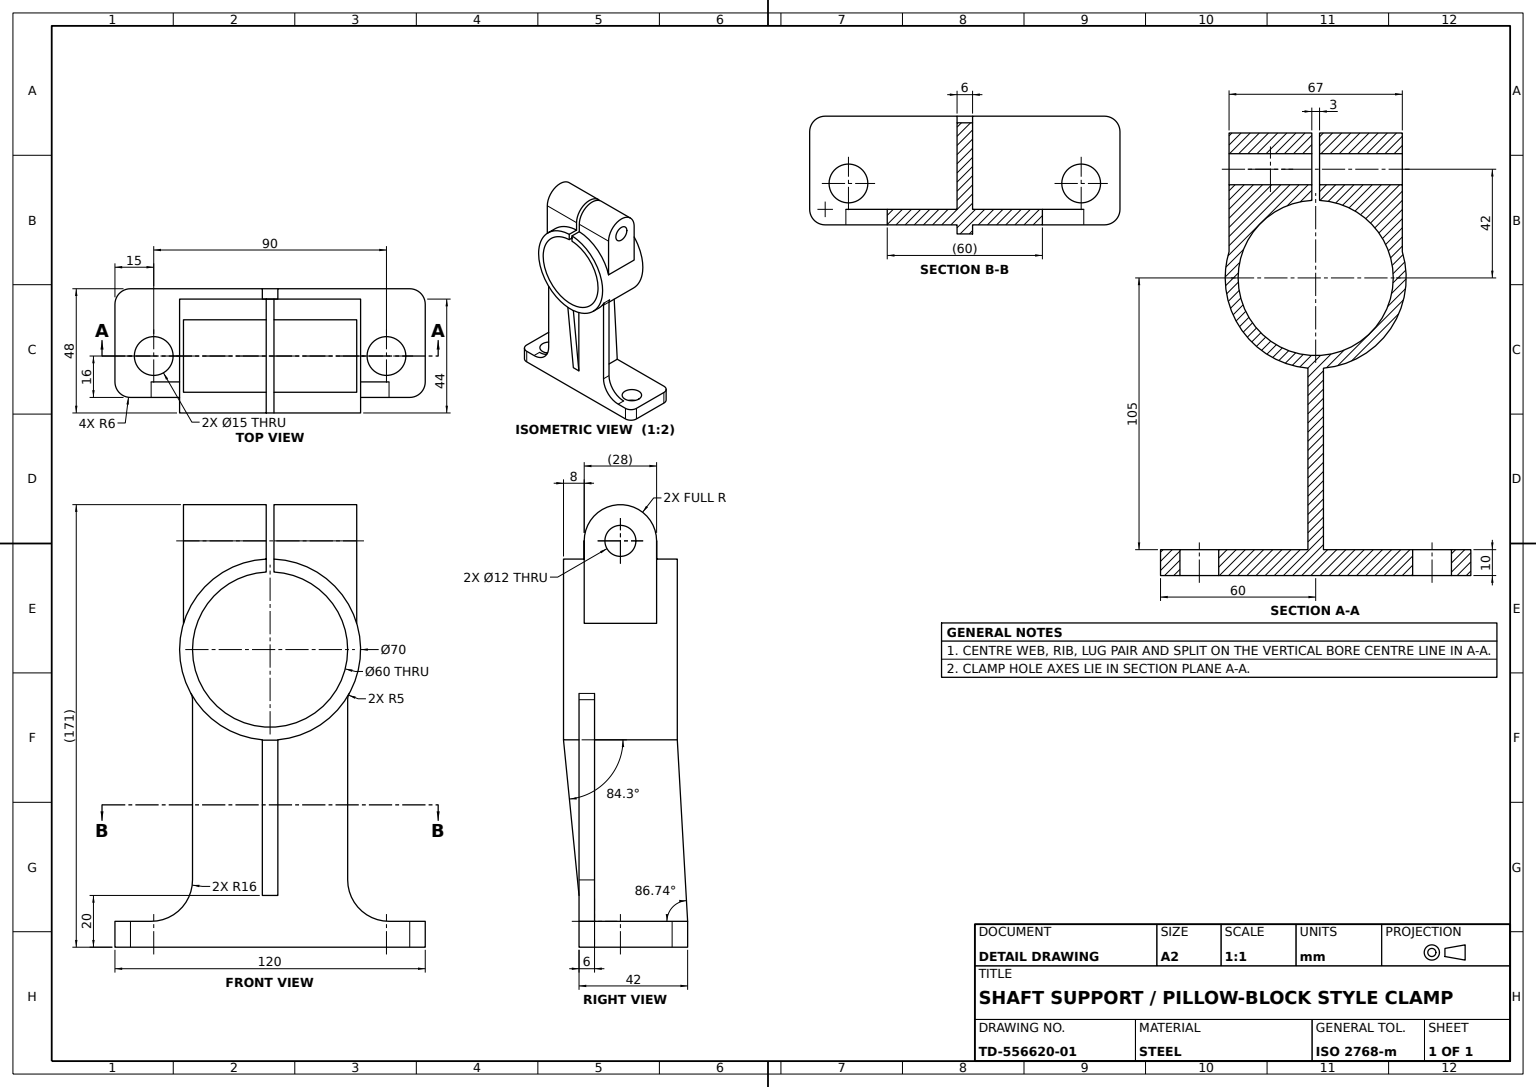
ISO-10303-21;
HEADER;
FILE_DESCRIPTION((''),'2;1');
FILE_NAME('','',(''),(''),'','','');
FILE_SCHEMA(('AUTOMOTIVE_DESIGN'));
ENDSEC;
DATA;
#1=APPLICATION_CONTEXT('');
#2=PRODUCT_CONTEXT('',#1,'mechanical');
#3=PRODUCT('','','',(#2));
#4=PRODUCT_DEFINITION_FORMATION('','',#3);
#5=PRODUCT_DEFINITION_CONTEXT('',#1,'design');
#6=PRODUCT_DEFINITION('','',#4,#5);
#7=PRODUCT_DEFINITION_SHAPE('','',#6);
#8=(LENGTH_UNIT()NAMED_UNIT(*)SI_UNIT(.MILLI.,.METRE.));
#9=(NAMED_UNIT(*)PLANE_ANGLE_UNIT()SI_UNIT($,.RADIAN.));
#10=(NAMED_UNIT(*)SI_UNIT($,.STERADIAN.)SOLID_ANGLE_UNIT());
#11=UNCERTAINTY_MEASURE_WITH_UNIT(LENGTH_MEASURE(1.E-05),#8,'distance_accuracy_value','');
#12=(GEOMETRIC_REPRESENTATION_CONTEXT(3)GLOBAL_UNCERTAINTY_ASSIGNED_CONTEXT((#11))GLOBAL_UNIT_ASSIGNED_CONTEXT((#8,#9,#10))REPRESENTATION_CONTEXT('',''));
#13=CARTESIAN_POINT('',(14.,34.967842,-1.5));
#14=VERTEX_POINT('',#13);
#15=CARTESIAN_POINT('',(22.,34.967842,-1.5));
#16=VERTEX_POINT('',#15);
#17=DIRECTION('',(1.,0.,0.));
#18=VECTOR('',#17,1000.);
#19=LINE('',#15,#18);
#20=EDGE_CURVE('',#14,#16,#19,.T.);
#21=ORIENTED_EDGE('',*,*,#20,.T.);
#22=CARTESIAN_POINT('',(22.,-34.871192,-3.));
#23=VERTEX_POINT('',#22);
#24=CARTESIAN_POINT('',(22.,0.,0.));
#25=DIRECTION('',(0.,0.,-1.));
#26=AXIS2_PLACEMENT_3D('',#24,#17,#25);
#27=CIRCLE('',#26,35.);
#28=EDGE_CURVE('',#23,#16,#27,.T.);
#29=ORIENTED_EDGE('',*,*,#28,.F.);
#30=CARTESIAN_POINT('',(16.,-34.871192,-3.));
#31=VERTEX_POINT('',#30);
#32=LINE('',#22,#18);
#33=EDGE_CURVE('',#31,#23,#32,.T.);
#34=ORIENTED_EDGE('',*,*,#33,.F.);
#35=CARTESIAN_POINT('',(16.,-16.944302,-30.625));
#36=VERTEX_POINT('',#35);
#37=CARTESIAN_POINT('',(16.,0.,0.));
#38=DIRECTION('',(-1.,0.,0.));
#39=AXIS2_PLACEMENT_3D('',#37,#38,#25);
#40=CIRCLE('',#39,35.);
#41=EDGE_CURVE('',#36,#31,#40,.T.);
#42=ORIENTED_EDGE('',*,*,#41,.F.);
#43=CARTESIAN_POINT('',(10.,-16.944302,-30.625));
#44=VERTEX_POINT('',#43);
#45=CARTESIAN_POINT('',(22.,-16.944302,-30.625));
#46=VECTOR('',#38,1000.);
#47=LINE('',#45,#46);
#48=EDGE_CURVE('',#36,#44,#47,.T.);
#49=ORIENTED_EDGE('',*,*,#48,.T.);
#50=CARTESIAN_POINT('',(10.,-34.871192,-3.));
#51=VERTEX_POINT('',#50);
#52=CARTESIAN_POINT('',(10.,0.,0.));
#53=AXIS2_PLACEMENT_3D('',#52,#38,#25);
#54=CIRCLE('',#53,35.);
#55=EDGE_CURVE('',#44,#51,#54,.T.);
#56=ORIENTED_EDGE('',*,*,#55,.T.);
#57=CARTESIAN_POINT('',(-22.,-34.871192,-3.));
#58=VERTEX_POINT('',#57);
#59=CARTESIAN_POINT('',(22.002,-34.871192,-3.));
#60=LINE('',#59,#46);
#61=EDGE_CURVE('',#51,#58,#60,.T.);
#62=ORIENTED_EDGE('',*,*,#61,.T.);
#63=CARTESIAN_POINT('',(-22.,34.967842,-1.5));
#64=VERTEX_POINT('',#63);
#65=CARTESIAN_POINT('',(-22.,0.,0.));
#66=AXIS2_PLACEMENT_3D('',#65,#17,#25);
#67=CIRCLE('',#66,35.);
#68=EDGE_CURVE('',#58,#64,#67,.T.);
#69=ORIENTED_EDGE('',*,*,#68,.T.);
#70=CARTESIAN_POINT('',(-14.,34.967842,-1.5));
#71=VERTEX_POINT('',#70);
#72=EDGE_CURVE('',#64,#71,#19,.T.);
#73=ORIENTED_EDGE('',*,*,#72,.T.);
#74=CARTESIAN_POINT('',(-14.,10.136567,-33.5));
#75=VERTEX_POINT('',#74);
#76=CARTESIAN_POINT('',(-14.,0.,0.));
#77=DIRECTION('',(0.,1.,0.));
#78=AXIS2_PLACEMENT_3D('',#76,#17,#77);
#79=CIRCLE('',#78,35.);
#80=EDGE_CURVE('',#75,#71,#79,.T.);
#81=ORIENTED_EDGE('',*,*,#80,.F.);
#82=CARTESIAN_POINT('',(14.,10.136567,-33.5));
#83=VERTEX_POINT('',#82);
#84=CARTESIAN_POINT('',(22.,10.136567,-33.5));
#85=LINE('',#84,#46);
#86=EDGE_CURVE('',#83,#75,#85,.T.);
#87=ORIENTED_EDGE('',*,*,#86,.F.);
#88=CARTESIAN_POINT('',(14.,0.,0.));
#89=DIRECTION('',(0.,0.,1.));
#90=AXIS2_PLACEMENT_3D('',#88,#38,#89);
#91=CIRCLE('',#90,35.);
#92=EDGE_CURVE('',#14,#83,#91,.T.);
#93=ORIENTED_EDGE('',*,*,#92,.F.);
#94=EDGE_LOOP('',(#21,#29,#34,#42,#49,#56,#62,#69,#73,#81,#87,#93));
#95=FACE_OUTER_BOUND('',#94,.T.);
#96=AXIS2_PLACEMENT_3D('',#24,#38,#89);
#97=CYLINDRICAL_SURFACE('',#96,35.);
#98=ADVANCED_FACE('',(#95),#97,.T.);
#99=CARTESIAN_POINT('',(0.,-115.,37.5));
#100=VERTEX_POINT('',#99);
#101=CARTESIAN_POINT('',(0.,-115.,52.5));
#102=VERTEX_POINT('',#101);
#103=CARTESIAN_POINT('',(0.,-115.,45.));
#104=DIRECTION('',(0.,-1.,0.));
#105=AXIS2_PLACEMENT_3D('',#103,#104,#89);
#106=CIRCLE('',#105,7.5);
#107=EDGE_CURVE('',#100,#102,#106,.T.);
#108=ORIENTED_EDGE('',*,*,#107,.F.);
#109=EDGE_CURVE('',#102,#100,#106,.T.);
#110=ORIENTED_EDGE('',*,*,#109,.F.);
#111=EDGE_LOOP('',(#108,#110));
#112=FACE_BOUND('',#111,.T.);
#113=CARTESIAN_POINT('',(-20.,-115.,60.));
#114=VERTEX_POINT('',#113);
#115=CARTESIAN_POINT('',(-26.,-115.,54.));
#116=VERTEX_POINT('',#115);
#117=CARTESIAN_POINT('',(-20.,-115.,54.));
#118=AXIS2_PLACEMENT_3D('',#117,#104,#89);
#119=CIRCLE('',#118,6.);
#120=EDGE_CURVE('',#114,#116,#119,.T.);
#121=ORIENTED_EDGE('',*,*,#120,.T.);
#122=CARTESIAN_POINT('',(-26.,-115.,-54.));
#123=VERTEX_POINT('',#122);
#124=CARTESIAN_POINT('',(-26.,-115.,-60.));
#125=VECTOR('',#89,1000.);
#126=LINE('',#124,#125);
#127=EDGE_CURVE('',#123,#116,#126,.T.);
#128=ORIENTED_EDGE('',*,*,#127,.F.);
#129=CARTESIAN_POINT('',(-20.,-115.,-60.));
#130=VERTEX_POINT('',#129);
#131=CARTESIAN_POINT('',(-20.,-115.,-54.));
#132=AXIS2_PLACEMENT_3D('',#131,#104,#89);
#133=CIRCLE('',#132,6.);
#134=EDGE_CURVE('',#123,#130,#133,.T.);
#135=ORIENTED_EDGE('',*,*,#134,.T.);
#136=CARTESIAN_POINT('',(10.,-115.,-60.));
#137=VERTEX_POINT('',#136);
#138=LINE('',#124,#46);
#139=EDGE_CURVE('',#137,#130,#138,.T.);
#140=ORIENTED_EDGE('',*,*,#139,.F.);
#141=CARTESIAN_POINT('',(16.,-115.,-54.));
#142=VERTEX_POINT('',#141);
#143=CARTESIAN_POINT('',(10.,-115.,-54.));
#144=AXIS2_PLACEMENT_3D('',#143,#104,#89);
#145=CIRCLE('',#144,6.);
#146=EDGE_CURVE('',#137,#142,#145,.T.);
#147=ORIENTED_EDGE('',*,*,#146,.T.);
#148=CARTESIAN_POINT('',(16.,-115.,54.));
#149=VERTEX_POINT('',#148);
#150=CARTESIAN_POINT('',(16.,-115.,-60.));
#151=VECTOR('',#25,1000.);
#152=LINE('',#150,#151);
#153=EDGE_CURVE('',#149,#142,#152,.T.);
#154=ORIENTED_EDGE('',*,*,#153,.F.);
#155=CARTESIAN_POINT('',(10.,-115.,60.));
#156=VERTEX_POINT('',#155);
#157=CARTESIAN_POINT('',(10.,-115.,54.));
#158=AXIS2_PLACEMENT_3D('',#157,#104,#89);
#159=CIRCLE('',#158,6.);
#160=EDGE_CURVE('',#149,#156,#159,.T.);
#161=ORIENTED_EDGE('',*,*,#160,.T.);
#162=CARTESIAN_POINT('',(-26.,-115.,60.));
#163=LINE('',#162,#18);
#164=EDGE_CURVE('',#114,#156,#163,.T.);
#165=ORIENTED_EDGE('',*,*,#164,.F.);
#166=EDGE_LOOP('',(#121,#128,#135,#140,#147,#154,#161,#165));
#167=FACE_OUTER_BOUND('',#166,.T.);
#168=CARTESIAN_POINT('',(0.,-115.,-37.5));
#169=VERTEX_POINT('',#168);
#170=CARTESIAN_POINT('',(0.,-115.,-52.5));
#171=VERTEX_POINT('',#170);
#172=CARTESIAN_POINT('',(0.,-115.,-45.));
#173=AXIS2_PLACEMENT_3D('',#172,#104,#89);
#174=CIRCLE('',#173,7.5);
#175=EDGE_CURVE('',#169,#171,#174,.T.);
#176=ORIENTED_EDGE('',*,*,#175,.F.);
#177=EDGE_CURVE('',#171,#169,#174,.T.);
#178=ORIENTED_EDGE('',*,*,#177,.F.);
#179=EDGE_LOOP('',(#176,#178));
#180=FACE_BOUND('',#179,.T.);
#181=CARTESIAN_POINT('',(0.,-115.,0.));
#182=AXIS2_PLACEMENT_3D('',#181,#77,#89);
#183=PLANE('',#182);
#184=ADVANCED_FACE('',(#112,#167,#180),#183,.F.);
#185=ORIENTED_EDGE('',*,*,#33,.T.);
#186=CARTESIAN_POINT('',(22.,-35.,-3.));
#187=VERTEX_POINT('',#186);
#188=CARTESIAN_POINT('',(22.,-40.,-3.));
#189=VECTOR('',#77,1000.);
#190=LINE('',#188,#189);
#191=EDGE_CURVE('',#187,#23,#190,.T.);
#192=ORIENTED_EDGE('',*,*,#191,.F.);
#193=CARTESIAN_POINT('',(16.,-95.,-3.));
#194=VERTEX_POINT('',#193);
#195=DIRECTION('',(0.099503719,0.99503719,0.));
#196=VECTOR('',#195,1000.);
#197=LINE('',#193,#196);
#198=EDGE_CURVE('',#194,#187,#197,.T.);
#199=ORIENTED_EDGE('',*,*,#198,.F.);
#200=CARTESIAN_POINT('',(16.,0.,-3.));
#201=VECTOR('',#104,1000.);
#202=LINE('',#200,#201);
#203=EDGE_CURVE('',#31,#194,#202,.T.);
#204=ORIENTED_EDGE('',*,*,#203,.F.);
#205=EDGE_LOOP('',(#185,#192,#199,#204));
#206=FACE_OUTER_BOUND('',#205,.T.);
#207=CARTESIAN_POINT('',(-2.,-40.,-3.));
#208=AXIS2_PLACEMENT_3D('',#207,#89,#17);
#209=PLANE('',#208);
#210=ADVANCED_FACE('',(#206),#209,.F.);
#211=CARTESIAN_POINT('',(0.,-105.,52.5));
#212=VERTEX_POINT('',#211);
#213=CARTESIAN_POINT('',(0.,-105.,37.5));
#214=VERTEX_POINT('',#213);
#215=CARTESIAN_POINT('',(0.,-105.,45.));
#216=AXIS2_PLACEMENT_3D('',#215,#77,#89);
#217=CIRCLE('',#216,7.5);
#218=EDGE_CURVE('',#212,#214,#217,.T.);
#219=ORIENTED_EDGE('',*,*,#218,.F.);
#220=EDGE_CURVE('',#214,#212,#217,.T.);
#221=ORIENTED_EDGE('',*,*,#220,.F.);
#222=EDGE_LOOP('',(#219,#221));
#223=FACE_BOUND('',#222,.T.);
#224=CARTESIAN_POINT('',(10.,-105.,60.));
#225=VERTEX_POINT('',#224);
#226=CARTESIAN_POINT('',(16.,-105.,54.));
#227=VERTEX_POINT('',#226);
#228=CARTESIAN_POINT('',(10.,-105.,54.));
#229=AXIS2_PLACEMENT_3D('',#228,#77,#89);
#230=CIRCLE('',#229,6.);
#231=EDGE_CURVE('',#225,#227,#230,.T.);
#232=ORIENTED_EDGE('',*,*,#231,.T.);
#233=CARTESIAN_POINT('',(16.,-105.,46.));
#234=VERTEX_POINT('',#233);
#235=CARTESIAN_POINT('',(16.,-105.,-60.));
#236=LINE('',#235,#151);
#237=EDGE_CURVE('',#227,#234,#236,.T.);
#238=ORIENTED_EDGE('',*,*,#237,.T.);
#239=CARTESIAN_POINT('',(10.,-105.,46.));
#240=VERTEX_POINT('',#239);
#241=LINE('',#239,#46);
#242=EDGE_CURVE('',#234,#240,#241,.T.);
#243=ORIENTED_EDGE('',*,*,#242,.T.);
#244=CARTESIAN_POINT('',(10.,-105.,3.));
#245=VERTEX_POINT('',#244);
#246=CARTESIAN_POINT('',(10.,-105.,30.));
#247=LINE('',#246,#151);
#248=EDGE_CURVE('',#240,#245,#247,.T.);
#249=ORIENTED_EDGE('',*,*,#248,.T.);
#250=CARTESIAN_POINT('',(-26.,-105.,3.));
#251=VERTEX_POINT('',#250);
#252=CARTESIAN_POINT('',(22.002,-105.,3.));
#253=LINE('',#252,#46);
#254=EDGE_CURVE('',#245,#251,#253,.T.);
#255=ORIENTED_EDGE('',*,*,#254,.T.);
#256=CARTESIAN_POINT('',(-26.,-105.,54.));
#257=VERTEX_POINT('',#256);
#258=CARTESIAN_POINT('',(-26.,-105.,-60.));
#259=LINE('',#258,#125);
#260=EDGE_CURVE('',#251,#257,#259,.T.);
#261=ORIENTED_EDGE('',*,*,#260,.T.);
#262=CARTESIAN_POINT('',(-20.,-105.,60.));
#263=VERTEX_POINT('',#262);
#264=CARTESIAN_POINT('',(-20.,-105.,54.));
#265=AXIS2_PLACEMENT_3D('',#264,#77,#89);
#266=CIRCLE('',#265,6.);
#267=EDGE_CURVE('',#257,#263,#266,.T.);
#268=ORIENTED_EDGE('',*,*,#267,.T.);
#269=CARTESIAN_POINT('',(-26.,-105.,60.));
#270=LINE('',#269,#18);
#271=EDGE_CURVE('',#263,#225,#270,.T.);
#272=ORIENTED_EDGE('',*,*,#271,.T.);
#273=EDGE_LOOP('',(#232,#238,#243,#249,#255,#261,#268,#272));
#274=FACE_OUTER_BOUND('',#273,.T.);
#275=CARTESIAN_POINT('',(0.,-105.,0.));
#276=AXIS2_PLACEMENT_3D('',#275,#77,#89);
#277=PLANE('',#276);
#278=ADVANCED_FACE('',(#223,#274),#277,.T.);
#279=CARTESIAN_POINT('',(14.,42.,33.5));
#280=VERTEX_POINT('',#279);
#281=CARTESIAN_POINT('',(14.,42.,1.5));
#282=VERTEX_POINT('',#281);
#283=LINE('',#279,#151);
#284=EDGE_CURVE('',#280,#282,#283,.T.);
#285=ORIENTED_EDGE('',*,*,#284,.F.);
#286=CARTESIAN_POINT('',(14.,10.136567,33.5));
#287=VERTEX_POINT('',#286);
#288=LINE('',#279,#189);
#289=EDGE_CURVE('',#287,#280,#288,.T.);
#290=ORIENTED_EDGE('',*,*,#289,.F.);
#291=CARTESIAN_POINT('',(14.,34.967842,1.5));
#292=VERTEX_POINT('',#291);
#293=EDGE_CURVE('',#287,#292,#91,.T.);
#294=ORIENTED_EDGE('',*,*,#293,.T.);
#295=LINE('',#281,#189);
#296=EDGE_CURVE('',#292,#282,#295,.T.);
#297=ORIENTED_EDGE('',*,*,#296,.T.);
#298=EDGE_LOOP('',(#285,#290,#294,#297));
#299=FACE_OUTER_BOUND('',#298,.T.);
#300=AXIS2_PLACEMENT_3D('',#279,#38,#89);
#301=PLANE('',#300);
#302=ADVANCED_FACE('',(#299),#301,.F.);
#303=CARTESIAN_POINT('',(16.,-95.,3.));
#304=VERTEX_POINT('',#303);
#305=CARTESIAN_POINT('',(16.,-95.,0.));
#306=LINE('',#305,#151);
#307=EDGE_CURVE('',#304,#194,#306,.T.);
#308=ORIENTED_EDGE('',*,*,#307,.T.);
#309=ORIENTED_EDGE('',*,*,#198,.T.);
#310=CARTESIAN_POINT('',(22.,-35.,3.));
#311=VERTEX_POINT('',#310);
#312=CARTESIAN_POINT('',(22.,-35.,0.));
#313=LINE('',#312,#125);
#314=EDGE_CURVE('',#187,#311,#313,.T.);
#315=ORIENTED_EDGE('',*,*,#314,.T.);
#316=LINE('',#303,#196);
#317=EDGE_CURVE('',#304,#311,#316,.T.);
#318=ORIENTED_EDGE('',*,*,#317,.F.);
#319=EDGE_LOOP('',(#308,#309,#315,#318));
#320=FACE_OUTER_BOUND('',#319,.T.);
#321=DIRECTION('',(0.99503719,-0.099503719,0.));
#322=AXIS2_PLACEMENT_3D('',#305,#321,#195);
#323=PLANE('',#322);
#324=ADVANCED_FACE('',(#320),#323,.T.);
#325=CARTESIAN_POINT('',(10.,-105.,-46.));
#326=VERTEX_POINT('',#325);
#327=CARTESIAN_POINT('',(16.,-105.,-46.));
#328=VERTEX_POINT('',#327);
#329=LINE('',#327,#18);
#330=EDGE_CURVE('',#326,#328,#329,.T.);
#331=ORIENTED_EDGE('',*,*,#330,.F.);
#332=CARTESIAN_POINT('',(10.,-89.,-30.));
#333=VERTEX_POINT('',#332);
#334=CARTESIAN_POINT('',(10.,-89.,-46.));
#335=AXIS2_PLACEMENT_3D('',#334,#17,#25);
#336=CIRCLE('',#335,16.);
#337=EDGE_CURVE('',#333,#326,#336,.T.);
#338=ORIENTED_EDGE('',*,*,#337,.F.);
#339=CARTESIAN_POINT('',(16.,-89.,-30.));
#340=VERTEX_POINT('',#339);
#341=LINE('',#332,#46);
#342=EDGE_CURVE('',#340,#333,#341,.T.);
#343=ORIENTED_EDGE('',*,*,#342,.F.);
#344=CARTESIAN_POINT('',(16.,-89.,-46.));
#345=AXIS2_PLACEMENT_3D('',#344,#38,#25);
#346=CIRCLE('',#345,16.);
#347=EDGE_CURVE('',#328,#340,#346,.T.);
#348=ORIENTED_EDGE('',*,*,#347,.F.);
#349=EDGE_LOOP('',(#331,#338,#343,#348));
#350=FACE_OUTER_BOUND('',#349,.T.);
#351=CARTESIAN_POINT('',(0.,-89.,-46.));
#352=AXIS2_PLACEMENT_3D('',#351,#38,#89);
#353=CYLINDRICAL_SURFACE('',#352,16.);
#354=ADVANCED_FACE('',(#350),#353,.F.);
#355=CARTESIAN_POINT('',(-26.,-105.,-3.));
#356=VERTEX_POINT('',#355);
#357=DIRECTION('',(0.056945345,0.998377297,0.));
#358=VECTOR('',#357,1000.);
#359=LINE('',#57,#358);
#360=EDGE_CURVE('',#356,#58,#359,.T.);
#361=ORIENTED_EDGE('',*,*,#360,.F.);
#362=CARTESIAN_POINT('',(-26.,-105.,-60.001));
#363=LINE('',#362,#125);
#364=EDGE_CURVE('',#356,#251,#363,.T.);
#365=ORIENTED_EDGE('',*,*,#364,.T.);
#366=CARTESIAN_POINT('',(-22.,-34.871192,3.));
#367=VERTEX_POINT('',#366);
#368=LINE('',#366,#358);
#369=EDGE_CURVE('',#251,#367,#368,.T.);
#370=ORIENTED_EDGE('',*,*,#369,.T.);
#371=CARTESIAN_POINT('',(-22.009814,-35.043253,1.));
#372=CARTESIAN_POINT('',(-22.009814,-35.043253,-1.));
#373=B_SPLINE_CURVE_WITH_KNOTS('',3,(#366,#371,#372,#57),.UNSPECIFIED.,.F.,.F.,(4,4),(0.,1.),.UNSPECIFIED.);
#374=EDGE_CURVE('',#367,#58,#373,.T.);
#375=ORIENTED_EDGE('',*,*,#374,.T.);
#376=EDGE_LOOP('',(#361,#365,#370,#375));
#377=FACE_OUTER_BOUND('',#376,.T.);
#378=CARTESIAN_POINT('',(-22.,-34.871192,-60.001));
#379=DIRECTION('',(0.998377297,-0.056945345,0.));
#380=AXIS2_PLACEMENT_3D('',#378,#379,#357);
#381=PLANE('',#380);
#382=ADVANCED_FACE('',(#377),#381,.F.);
#383=ORIENTED_EDGE('',*,*,#342,.T.);
#384=CARTESIAN_POINT('',(10.,-19.364917,-30.));
#385=VERTEX_POINT('',#384);
#386=CARTESIAN_POINT('',(10.,-105.,-30.));
#387=LINE('',#386,#189);
#388=EDGE_CURVE('',#333,#385,#387,.T.);
#389=ORIENTED_EDGE('',*,*,#388,.T.);
#390=CARTESIAN_POINT('',(16.,-19.364917,-30.));
#391=VERTEX_POINT('',#390);
#392=LINE('',#384,#18);
#393=EDGE_CURVE('',#385,#391,#392,.T.);
#394=ORIENTED_EDGE('',*,*,#393,.T.);
#395=CARTESIAN_POINT('',(16.,-105.,-30.));
#396=LINE('',#395,#189);
#397=EDGE_CURVE('',#340,#391,#396,.T.);
#398=ORIENTED_EDGE('',*,*,#397,.F.);
#399=EDGE_LOOP('',(#383,#389,#394,#398));
#400=FACE_OUTER_BOUND('',#399,.T.);
#401=AXIS2_PLACEMENT_3D('',#386,#25,#38);
#402=PLANE('',#401);
#403=ADVANCED_FACE('',(#400),#402,.T.);
#404=CARTESIAN_POINT('',(-22.,0.,30.));
#405=VERTEX_POINT('',#404);
#406=CARTESIAN_POINT('',(-22.,0.,-30.));
#407=VERTEX_POINT('',#406);
#408=CIRCLE('',#66,30.);
#409=EDGE_CURVE('',#405,#407,#408,.T.);
#410=ORIENTED_EDGE('',*,*,#409,.T.);
#411=CARTESIAN_POINT('',(-22.,29.962477,-1.5));
#412=VERTEX_POINT('',#411);
#413=EDGE_CURVE('',#407,#412,#408,.T.);
#414=ORIENTED_EDGE('',*,*,#413,.T.);
#415=CARTESIAN_POINT('',(-22.,0.,-1.5));
#416=LINE('',#415,#189);
#417=EDGE_CURVE('',#412,#64,#416,.T.);
#418=ORIENTED_EDGE('',*,*,#417,.T.);
#419=ORIENTED_EDGE('',*,*,#68,.F.);
#420=ORIENTED_EDGE('',*,*,#374,.F.);
#421=CARTESIAN_POINT('',(-22.,0.,35.));
#422=VERTEX_POINT('',#421);
#423=EDGE_CURVE('',#422,#367,#67,.T.);
#424=ORIENTED_EDGE('',*,*,#423,.F.);
#425=CARTESIAN_POINT('',(-22.,34.967842,1.5));
#426=VERTEX_POINT('',#425);
#427=EDGE_CURVE('',#426,#422,#67,.T.);
#428=ORIENTED_EDGE('',*,*,#427,.F.);
#429=CARTESIAN_POINT('',(-22.,29.962477,1.5));
#430=VERTEX_POINT('',#429);
#431=CARTESIAN_POINT('',(-22.,0.,1.5));
#432=LINE('',#431,#201);
#433=EDGE_CURVE('',#426,#430,#432,.T.);
#434=ORIENTED_EDGE('',*,*,#433,.T.);
#435=EDGE_CURVE('',#430,#405,#408,.T.);
#436=ORIENTED_EDGE('',*,*,#435,.T.);
#437=EDGE_LOOP('',(#410,#414,#418,#419,#420,#424,#428,#434,#436));
#438=FACE_OUTER_BOUND('',#437,.T.);
#439=PLANE('',#66);
#440=ADVANCED_FACE('',(#438),#439,.F.);
#441=CARTESIAN_POINT('',(-20.,-105.,-60.));
#442=VERTEX_POINT('',#441);
#443=LINE('',#129,#189);
#444=EDGE_CURVE('',#130,#442,#443,.T.);
#445=ORIENTED_EDGE('',*,*,#444,.F.);
#446=ORIENTED_EDGE('',*,*,#134,.F.);
#447=CARTESIAN_POINT('',(-26.,-105.,-54.));
#448=VERTEX_POINT('',#447);
#449=LINE('',#122,#201);
#450=EDGE_CURVE('',#448,#123,#449,.T.);
#451=ORIENTED_EDGE('',*,*,#450,.F.);
#452=CARTESIAN_POINT('',(-20.,-105.,-54.));
#453=AXIS2_PLACEMENT_3D('',#452,#77,#89);
#454=CIRCLE('',#453,6.);
#455=EDGE_CURVE('',#442,#448,#454,.T.);
#456=ORIENTED_EDGE('',*,*,#455,.F.);
#457=EDGE_LOOP('',(#445,#446,#451,#456));
#458=FACE_OUTER_BOUND('',#457,.T.);
#459=AXIS2_PLACEMENT_3D('',#131,#77,#89);
#460=CYLINDRICAL_SURFACE('',#459,6.);
#461=ADVANCED_FACE('',(#458),#460,.T.);
#462=ORIENTED_EDGE('',*,*,#360,.T.);
#463=ORIENTED_EDGE('',*,*,#61,.F.);
#464=CARTESIAN_POINT('',(10.,-105.,-3.));
#465=VERTEX_POINT('',#464);
#466=LINE('',#464,#201);
#467=EDGE_CURVE('',#51,#465,#466,.T.);
#468=ORIENTED_EDGE('',*,*,#467,.T.);
#469=CARTESIAN_POINT('',(22.002,-105.,-3.));
#470=LINE('',#469,#46);
#471=EDGE_CURVE('',#465,#356,#470,.T.);
#472=ORIENTED_EDGE('',*,*,#471,.T.);
#473=EDGE_LOOP('',(#462,#463,#468,#472));
#474=FACE_OUTER_BOUND('',#473,.T.);
#475=AXIS2_PLACEMENT_3D('',#469,#25,#38);
#476=PLANE('',#475);
#477=ADVANCED_FACE('',(#474),#476,.T.);
#478=CARTESIAN_POINT('',(-14.,42.,-1.5));
#479=VERTEX_POINT('',#478);
#480=CARTESIAN_POINT('',(-14.,42.,-33.5));
#481=VERTEX_POINT('',#480);
#482=CARTESIAN_POINT('',(-14.,42.,33.5));
#483=LINE('',#482,#151);
#484=EDGE_CURVE('',#479,#481,#483,.T.);
#485=ORIENTED_EDGE('',*,*,#484,.F.);
#486=CARTESIAN_POINT('',(14.,42.,-1.5));
#487=VERTEX_POINT('',#486);
#488=CARTESIAN_POINT('',(0.,42.,-1.5));
#489=AXIS2_PLACEMENT_3D('',#488,#25,#38);
#490=CIRCLE('',#489,14.);
#491=EDGE_CURVE('',#479,#487,#490,.T.);
#492=ORIENTED_EDGE('',*,*,#491,.T.);
#493=CARTESIAN_POINT('',(14.,42.,-33.5));
#494=VERTEX_POINT('',#493);
#495=EDGE_CURVE('',#487,#494,#283,.T.);
#496=ORIENTED_EDGE('',*,*,#495,.T.);
#497=CARTESIAN_POINT('',(0.,42.,-33.5));
#498=AXIS2_PLACEMENT_3D('',#497,#89,#17);
#499=CIRCLE('',#498,14.);
#500=EDGE_CURVE('',#494,#481,#499,.T.);
#501=ORIENTED_EDGE('',*,*,#500,.T.);
#502=EDGE_LOOP('',(#485,#492,#496,#501));
#503=FACE_OUTER_BOUND('',#502,.T.);
#504=CARTESIAN_POINT('',(0.,42.,33.5));
#505=AXIS2_PLACEMENT_3D('',#504,#25,#38);
#506=CYLINDRICAL_SURFACE('',#505,14.);
#507=ADVANCED_FACE('',(#503),#506,.T.);
#508=LINE('',#113,#201);
#509=EDGE_CURVE('',#263,#114,#508,.T.);
#510=ORIENTED_EDGE('',*,*,#509,.F.);
#511=ORIENTED_EDGE('',*,*,#267,.F.);
#512=LINE('',#115,#189);
#513=EDGE_CURVE('',#116,#257,#512,.T.);
#514=ORIENTED_EDGE('',*,*,#513,.F.);
#515=ORIENTED_EDGE('',*,*,#120,.F.);
#516=EDGE_LOOP('',(#510,#511,#514,#515));
#517=FACE_OUTER_BOUND('',#516,.T.);
#518=AXIS2_PLACEMENT_3D('',#117,#77,#89);
#519=CYLINDRICAL_SURFACE('',#518,6.);
#520=ADVANCED_FACE('',(#517),#519,.T.);
#521=CARTESIAN_POINT('',(10.,-105.,-60.));
#522=VERTEX_POINT('',#521);
#523=LINE('',#136,#201);
#524=EDGE_CURVE('',#522,#137,#523,.T.);
#525=ORIENTED_EDGE('',*,*,#524,.T.);
#526=ORIENTED_EDGE('',*,*,#139,.T.);
#527=ORIENTED_EDGE('',*,*,#444,.T.);
#528=LINE('',#258,#46);
#529=EDGE_CURVE('',#522,#442,#528,.T.);
#530=ORIENTED_EDGE('',*,*,#529,.F.);
#531=EDGE_LOOP('',(#525,#526,#527,#530));
#532=FACE_OUTER_BOUND('',#531,.T.);
#533=AXIS2_PLACEMENT_3D('',#124,#25,#38);
#534=PLANE('',#533);
#535=ADVANCED_FACE('',(#532),#534,.T.);
#536=CARTESIAN_POINT('',(10.,-34.871192,3.));
#537=VERTEX_POINT('',#536);
#538=LINE('',#244,#189);
#539=EDGE_CURVE('',#245,#537,#538,.T.);
#540=ORIENTED_EDGE('',*,*,#539,.T.);
#541=CARTESIAN_POINT('',(22.002,-34.871192,3.));
#542=LINE('',#541,#46);
#543=EDGE_CURVE('',#537,#367,#542,.T.);
#544=ORIENTED_EDGE('',*,*,#543,.T.);
#545=ORIENTED_EDGE('',*,*,#369,.F.);
#546=ORIENTED_EDGE('',*,*,#254,.F.);
#547=EDGE_LOOP('',(#540,#544,#545,#546));
#548=FACE_OUTER_BOUND('',#547,.T.);
#549=AXIS2_PLACEMENT_3D('',#252,#89,#17);
#550=PLANE('',#549);
#551=ADVANCED_FACE('',(#548),#550,.T.);
#552=CARTESIAN_POINT('',(22.,34.967842,1.5));
#553=VERTEX_POINT('',#552);
#554=CARTESIAN_POINT('',(22.,29.962477,1.5));
#555=VERTEX_POINT('',#554);
#556=CARTESIAN_POINT('',(22.,0.,1.5));
#557=LINE('',#556,#201);
#558=EDGE_CURVE('',#553,#555,#557,.T.);
#559=ORIENTED_EDGE('',*,*,#558,.T.);
#560=LINE('',#554,#46);
#561=EDGE_CURVE('',#555,#430,#560,.T.);
#562=ORIENTED_EDGE('',*,*,#561,.T.);
#563=ORIENTED_EDGE('',*,*,#433,.F.);
#564=CARTESIAN_POINT('',(-14.,34.967842,1.5));
#565=VERTEX_POINT('',#564);
#566=LINE('',#552,#46);
#567=EDGE_CURVE('',#565,#426,#566,.T.);
#568=ORIENTED_EDGE('',*,*,#567,.F.);
#569=CARTESIAN_POINT('',(-14.,42.,1.5));
#570=VERTEX_POINT('',#569);
#571=CARTESIAN_POINT('',(-14.,0.,1.5));
#572=LINE('',#571,#201);
#573=EDGE_CURVE('',#570,#565,#572,.T.);
#574=ORIENTED_EDGE('',*,*,#573,.F.);
#575=CARTESIAN_POINT('',(0.,42.,1.5));
#576=AXIS2_PLACEMENT_3D('',#575,#89,#17);
#577=CIRCLE('',#576,14.);
#578=EDGE_CURVE('',#282,#570,#577,.T.);
#579=ORIENTED_EDGE('',*,*,#578,.F.);
#580=ORIENTED_EDGE('',*,*,#296,.F.);
#581=EDGE_CURVE('',#553,#292,#566,.T.);
#582=ORIENTED_EDGE('',*,*,#581,.F.);
#583=EDGE_LOOP('',(#559,#562,#563,#568,#574,#579,#580,#582));
#584=FACE_OUTER_BOUND('',#583,.T.);
#585=CARTESIAN_POINT('',(6.,42.,1.5));
#586=VERTEX_POINT('',#585);
#587=CARTESIAN_POINT('',(-6.,42.,1.5));
#588=VERTEX_POINT('',#587);
#589=CIRCLE('',#576,6.);
#590=EDGE_CURVE('',#586,#588,#589,.T.);
#591=ORIENTED_EDGE('',*,*,#590,.T.);
#592=EDGE_CURVE('',#588,#586,#589,.T.);
#593=ORIENTED_EDGE('',*,*,#592,.T.);
#594=EDGE_LOOP('',(#591,#593));
#595=FACE_BOUND('',#594,.T.);
#596=CARTESIAN_POINT('',(-26.000025,0.,1.5));
#597=AXIS2_PLACEMENT_3D('',#596,#89,#17);
#598=PLANE('',#597);
#599=ADVANCED_FACE('',(#584,#595),#598,.F.);
#600=CARTESIAN_POINT('',(22.,29.962477,-1.5));
#601=VERTEX_POINT('',#600);
#602=CARTESIAN_POINT('',(22.,0.,-1.5));
#603=LINE('',#602,#189);
#604=EDGE_CURVE('',#601,#16,#603,.T.);
#605=ORIENTED_EDGE('',*,*,#604,.T.);
#606=ORIENTED_EDGE('',*,*,#20,.F.);
#607=LINE('',#486,#201);
#608=EDGE_CURVE('',#487,#14,#607,.T.);
#609=ORIENTED_EDGE('',*,*,#608,.F.);
#610=ORIENTED_EDGE('',*,*,#491,.F.);
#611=CARTESIAN_POINT('',(-14.,0.,-1.5));
#612=LINE('',#611,#189);
#613=EDGE_CURVE('',#71,#479,#612,.T.);
#614=ORIENTED_EDGE('',*,*,#613,.F.);
#615=ORIENTED_EDGE('',*,*,#72,.F.);
#616=ORIENTED_EDGE('',*,*,#417,.F.);
#617=LINE('',#600,#18);
#618=EDGE_CURVE('',#412,#601,#617,.T.);
#619=ORIENTED_EDGE('',*,*,#618,.T.);
#620=EDGE_LOOP('',(#605,#606,#609,#610,#614,#615,#616,#619));
#621=FACE_OUTER_BOUND('',#620,.T.);
#622=CARTESIAN_POINT('',(6.,42.,-1.5));
#623=VERTEX_POINT('',#622);
#624=CARTESIAN_POINT('',(-6.,42.,-1.5));
#625=VERTEX_POINT('',#624);
#626=CIRCLE('',#489,6.);
#627=EDGE_CURVE('',#623,#625,#626,.T.);
#628=ORIENTED_EDGE('',*,*,#627,.T.);
#629=EDGE_CURVE('',#625,#623,#626,.T.);
#630=ORIENTED_EDGE('',*,*,#629,.T.);
#631=EDGE_LOOP('',(#628,#630));
#632=FACE_BOUND('',#631,.T.);
#633=CARTESIAN_POINT('',(-26.000025,0.,-1.5));
#634=AXIS2_PLACEMENT_3D('',#633,#25,#38);
#635=PLANE('',#634);
#636=ADVANCED_FACE('',(#621,#632),#635,.F.);
#637=CARTESIAN_POINT('',(22.,0.,-30.));
#638=VERTEX_POINT('',#637);
#639=LINE('',#637,#46);
#640=EDGE_CURVE('',#638,#407,#639,.T.);
#641=ORIENTED_EDGE('',*,*,#640,.T.);
#642=ORIENTED_EDGE('',*,*,#409,.F.);
#643=CARTESIAN_POINT('',(22.,0.,30.));
#644=VERTEX_POINT('',#643);
#645=LINE('',#643,#46);
#646=EDGE_CURVE('',#644,#405,#645,.T.);
#647=ORIENTED_EDGE('',*,*,#646,.F.);
#648=CIRCLE('',#26,30.);
#649=EDGE_CURVE('',#644,#638,#648,.T.);
#650=ORIENTED_EDGE('',*,*,#649,.T.);
#651=EDGE_LOOP('',(#641,#642,#647,#650));
#652=FACE_OUTER_BOUND('',#651,.T.);
#653=CYLINDRICAL_SURFACE('',#96,30.);
#654=ADVANCED_FACE('',(#652),#653,.F.);
#655=VERTEX_POINT('',#482);
#656=EDGE_CURVE('',#655,#570,#483,.T.);
#657=ORIENTED_EDGE('',*,*,#656,.F.);
#658=AXIS2_PLACEMENT_3D('',#504,#89,#17);
#659=CIRCLE('',#658,14.);
#660=EDGE_CURVE('',#280,#655,#659,.T.);
#661=ORIENTED_EDGE('',*,*,#660,.F.);
#662=ORIENTED_EDGE('',*,*,#284,.T.);
#663=ORIENTED_EDGE('',*,*,#578,.T.);
#664=EDGE_LOOP('',(#657,#661,#662,#663));
#665=FACE_OUTER_BOUND('',#664,.T.);
#666=ADVANCED_FACE('',(#665),#506,.T.);
#667=ORIENTED_EDGE('',*,*,#590,.F.);
#668=CARTESIAN_POINT('',(6.,42.,33.5));
#669=VERTEX_POINT('',#668);
#670=LINE('',#668,#151);
#671=EDGE_CURVE('',#669,#586,#670,.T.);
#672=ORIENTED_EDGE('',*,*,#671,.F.);
#673=CARTESIAN_POINT('',(-6.,42.,33.5));
#674=VERTEX_POINT('',#673);
#675=CIRCLE('',#658,6.);
#676=EDGE_CURVE('',#669,#674,#675,.T.);
#677=ORIENTED_EDGE('',*,*,#676,.T.);
#678=LINE('',#673,#151);
#679=EDGE_CURVE('',#674,#588,#678,.T.);
#680=ORIENTED_EDGE('',*,*,#679,.T.);
#681=EDGE_LOOP('',(#667,#672,#677,#680));
#682=FACE_OUTER_BOUND('',#681,.T.);
#683=CYLINDRICAL_SURFACE('',#505,6.);
#684=ADVANCED_FACE('',(#682),#683,.F.);
#685=ORIENTED_EDGE('',*,*,#509,.T.);
#686=ORIENTED_EDGE('',*,*,#164,.T.);
#687=LINE('',#155,#189);
#688=EDGE_CURVE('',#156,#225,#687,.T.);
#689=ORIENTED_EDGE('',*,*,#688,.T.);
#690=ORIENTED_EDGE('',*,*,#271,.F.);
#691=EDGE_LOOP('',(#685,#686,#689,#690));
#692=FACE_OUTER_BOUND('',#691,.T.);
#693=AXIS2_PLACEMENT_3D('',#162,#89,#17);
#694=PLANE('',#693);
#695=ADVANCED_FACE('',(#692),#694,.T.);
#696=CARTESIAN_POINT('',(16.,-19.364917,30.));
#697=VERTEX_POINT('',#696);
#698=CARTESIAN_POINT('',(16.,-89.,30.));
#699=VERTEX_POINT('',#698);
#700=CARTESIAN_POINT('',(16.,-105.,30.));
#701=LINE('',#700,#201);
#702=EDGE_CURVE('',#697,#699,#701,.T.);
#703=ORIENTED_EDGE('',*,*,#702,.F.);
#704=CARTESIAN_POINT('',(10.,-19.364917,30.));
#705=VERTEX_POINT('',#704);
#706=LINE('',#704,#46);
#707=EDGE_CURVE('',#697,#705,#706,.T.);
#708=ORIENTED_EDGE('',*,*,#707,.T.);
#709=CARTESIAN_POINT('',(10.,-89.,30.));
#710=VERTEX_POINT('',#709);
#711=LINE('',#246,#201);
#712=EDGE_CURVE('',#705,#710,#711,.T.);
#713=ORIENTED_EDGE('',*,*,#712,.T.);
#714=LINE('',#698,#18);
#715=EDGE_CURVE('',#710,#699,#714,.T.);
#716=ORIENTED_EDGE('',*,*,#715,.T.);
#717=EDGE_LOOP('',(#703,#708,#713,#716));
#718=FACE_OUTER_BOUND('',#717,.T.);
#719=AXIS2_PLACEMENT_3D('',#246,#89,#17);
#720=PLANE('',#719);
#721=ADVANCED_FACE('',(#718),#720,.T.);
#722=ORIENTED_EDGE('',*,*,#567,.T.);
#723=ORIENTED_EDGE('',*,*,#427,.T.);
#724=CARTESIAN_POINT('',(22.,0.,35.));
#725=VERTEX_POINT('',#724);
#726=LINE('',#724,#46);
#727=EDGE_CURVE('',#725,#422,#726,.T.);
#728=ORIENTED_EDGE('',*,*,#727,.F.);
#729=EDGE_CURVE('',#553,#725,#27,.T.);
#730=ORIENTED_EDGE('',*,*,#729,.F.);
#731=ORIENTED_EDGE('',*,*,#581,.T.);
#732=ORIENTED_EDGE('',*,*,#293,.F.);
#733=CARTESIAN_POINT('',(-14.,10.136567,33.5));
#734=VERTEX_POINT('',#733);
#735=CARTESIAN_POINT('',(22.,10.136567,33.5));
#736=LINE('',#735,#46);
#737=EDGE_CURVE('',#287,#734,#736,.T.);
#738=ORIENTED_EDGE('',*,*,#737,.T.);
#739=EDGE_CURVE('',#565,#734,#79,.T.);
#740=ORIENTED_EDGE('',*,*,#739,.F.);
#741=EDGE_LOOP('',(#722,#723,#728,#730,#731,#732,#738,#740));
#742=FACE_OUTER_BOUND('',#741,.T.);
#743=ADVANCED_FACE('',(#742),#97,.T.);
#744=CARTESIAN_POINT('',(16.,-16.944302,30.625));
#745=VERTEX_POINT('',#744);
#746=CARTESIAN_POINT('',(16.,-19.364917,35.));
#747=AXIS2_PLACEMENT_3D('',#746,#38,#25);
#748=CIRCLE('',#747,5.);
#749=EDGE_CURVE('',#745,#697,#748,.T.);
#750=ORIENTED_EDGE('',*,*,#749,.F.);
#751=CARTESIAN_POINT('',(10.,-16.944302,30.625));
#752=VERTEX_POINT('',#751);
#753=CARTESIAN_POINT('',(22.,-16.944302,30.625));
#754=LINE('',#753,#18);
#755=EDGE_CURVE('',#752,#745,#754,.T.);
#756=ORIENTED_EDGE('',*,*,#755,.F.);
#757=CARTESIAN_POINT('',(10.,-19.364917,35.));
#758=AXIS2_PLACEMENT_3D('',#757,#17,#25);
#759=CIRCLE('',#758,5.);
#760=EDGE_CURVE('',#705,#752,#759,.T.);
#761=ORIENTED_EDGE('',*,*,#760,.F.);
#762=ORIENTED_EDGE('',*,*,#707,.F.);
#763=EDGE_LOOP('',(#750,#756,#761,#762));
#764=FACE_OUTER_BOUND('',#763,.T.);
#765=CARTESIAN_POINT('',(22.,-19.364917,35.));
#766=AXIS2_PLACEMENT_3D('',#765,#38,#89);
#767=CYLINDRICAL_SURFACE('',#766,5.);
#768=ADVANCED_FACE('',(#764),#767,.F.);
#769=ORIENTED_EDGE('',*,*,#679,.F.);
#770=EDGE_CURVE('',#674,#669,#675,.T.);
#771=ORIENTED_EDGE('',*,*,#770,.T.);
#772=ORIENTED_EDGE('',*,*,#671,.T.);
#773=ORIENTED_EDGE('',*,*,#592,.F.);
#774=EDGE_LOOP('',(#769,#771,#772,#773));
#775=FACE_OUTER_BOUND('',#774,.T.);
#776=ADVANCED_FACE('',(#775),#683,.F.);
#777=CARTESIAN_POINT('',(10.,-89.,46.));
#778=AXIS2_PLACEMENT_3D('',#777,#17,#25);
#779=CIRCLE('',#778,16.);
#780=EDGE_CURVE('',#240,#710,#779,.T.);
#781=ORIENTED_EDGE('',*,*,#780,.T.);
#782=ORIENTED_EDGE('',*,*,#712,.F.);
#783=ORIENTED_EDGE('',*,*,#760,.T.);
#784=EDGE_CURVE('',#537,#752,#54,.T.);
#785=ORIENTED_EDGE('',*,*,#784,.F.);
#786=ORIENTED_EDGE('',*,*,#539,.F.);
#787=ORIENTED_EDGE('',*,*,#248,.F.);
#788=EDGE_LOOP('',(#781,#782,#783,#785,#786,#787));
#789=FACE_OUTER_BOUND('',#788,.T.);
#790=AXIS2_PLACEMENT_3D('',#52,#17,#25);
#791=PLANE('',#790);
#792=ADVANCED_FACE('',(#789),#791,.F.);
#793=CARTESIAN_POINT('',(6.,42.,-33.5));
#794=VERTEX_POINT('',#793);
#795=CARTESIAN_POINT('',(-6.,42.,-33.5));
#796=VERTEX_POINT('',#795);
#797=CIRCLE('',#498,6.);
#798=EDGE_CURVE('',#794,#796,#797,.T.);
#799=ORIENTED_EDGE('',*,*,#798,.F.);
#800=EDGE_CURVE('',#623,#794,#670,.T.);
#801=ORIENTED_EDGE('',*,*,#800,.F.);
#802=ORIENTED_EDGE('',*,*,#629,.F.);
#803=EDGE_CURVE('',#625,#796,#678,.T.);
#804=ORIENTED_EDGE('',*,*,#803,.T.);
#805=EDGE_LOOP('',(#799,#801,#802,#804));
#806=FACE_OUTER_BOUND('',#805,.T.);
#807=ADVANCED_FACE('',(#806),#683,.F.);
#808=ORIENTED_EDGE('',*,*,#798,.T.);
#809=EDGE_CURVE('',#796,#794,#797,.T.);
#810=ORIENTED_EDGE('',*,*,#809,.T.);
#811=EDGE_LOOP('',(#808,#810));
#812=FACE_BOUND('',#811,.T.);
#813=CARTESIAN_POINT('',(-14.,0.,-33.5));
#814=LINE('',#813,#201);
#815=EDGE_CURVE('',#481,#75,#814,.T.);
#816=ORIENTED_EDGE('',*,*,#815,.F.);
#817=ORIENTED_EDGE('',*,*,#500,.F.);
#818=LINE('',#493,#189);
#819=EDGE_CURVE('',#83,#494,#818,.T.);
#820=ORIENTED_EDGE('',*,*,#819,.F.);
#821=ORIENTED_EDGE('',*,*,#86,.T.);
#822=EDGE_LOOP('',(#816,#817,#820,#821));
#823=FACE_OUTER_BOUND('',#822,.T.);
#824=PLANE('',#498);
#825=ADVANCED_FACE('',(#812,#823),#824,.F.);
#826=ORIENTED_EDGE('',*,*,#127,.T.);
#827=ORIENTED_EDGE('',*,*,#513,.T.);
#828=ORIENTED_EDGE('',*,*,#260,.F.);
#829=ORIENTED_EDGE('',*,*,#364,.F.);
#830=EDGE_CURVE('',#448,#356,#259,.T.);
#831=ORIENTED_EDGE('',*,*,#830,.F.);
#832=ORIENTED_EDGE('',*,*,#450,.T.);
#833=EDGE_LOOP('',(#826,#827,#828,#829,#831,#832));
#834=FACE_OUTER_BOUND('',#833,.T.);
#835=AXIS2_PLACEMENT_3D('',#124,#38,#89);
#836=PLANE('',#835);
#837=ADVANCED_FACE('',(#834),#836,.T.);
#838=ORIENTED_EDGE('',*,*,#608,.T.);
#839=ORIENTED_EDGE('',*,*,#92,.T.);
#840=ORIENTED_EDGE('',*,*,#819,.T.);
#841=ORIENTED_EDGE('',*,*,#495,.F.);
#842=EDGE_LOOP('',(#838,#839,#840,#841));
#843=FACE_OUTER_BOUND('',#842,.T.);
#844=ADVANCED_FACE('',(#843),#301,.F.);
#845=CARTESIAN_POINT('',(16.,-89.,46.));
#846=AXIS2_PLACEMENT_3D('',#845,#38,#25);
#847=CIRCLE('',#846,16.);
#848=EDGE_CURVE('',#699,#234,#847,.T.);
#849=ORIENTED_EDGE('',*,*,#848,.T.);
#850=ORIENTED_EDGE('',*,*,#237,.F.);
#851=CARTESIAN_POINT('',(16.,0.,54.));
#852=LINE('',#851,#201);
#853=EDGE_CURVE('',#227,#149,#852,.T.);
#854=ORIENTED_EDGE('',*,*,#853,.T.);
#855=ORIENTED_EDGE('',*,*,#153,.T.);
#856=CARTESIAN_POINT('',(16.,-105.,-54.));
#857=VERTEX_POINT('',#856);
#858=CARTESIAN_POINT('',(16.,0.,-54.));
#859=LINE('',#858,#189);
#860=EDGE_CURVE('',#142,#857,#859,.T.);
#861=ORIENTED_EDGE('',*,*,#860,.T.);
#862=EDGE_CURVE('',#328,#857,#236,.T.);
#863=ORIENTED_EDGE('',*,*,#862,.F.);
#864=ORIENTED_EDGE('',*,*,#347,.T.);
#865=ORIENTED_EDGE('',*,*,#397,.T.);
#866=CARTESIAN_POINT('',(16.,-19.364917,-35.));
#867=AXIS2_PLACEMENT_3D('',#866,#38,#25);
#868=CIRCLE('',#867,5.);
#869=EDGE_CURVE('',#391,#36,#868,.T.);
#870=ORIENTED_EDGE('',*,*,#869,.T.);
#871=ORIENTED_EDGE('',*,*,#41,.T.);
#872=ORIENTED_EDGE('',*,*,#203,.T.);
#873=ORIENTED_EDGE('',*,*,#307,.F.);
#874=CARTESIAN_POINT('',(16.,-34.871192,3.));
#875=VERTEX_POINT('',#874);
#876=CARTESIAN_POINT('',(16.,0.,3.));
#877=LINE('',#876,#201);
#878=EDGE_CURVE('',#875,#304,#877,.T.);
#879=ORIENTED_EDGE('',*,*,#878,.F.);
#880=EDGE_CURVE('',#875,#745,#40,.T.);
#881=ORIENTED_EDGE('',*,*,#880,.T.);
#882=ORIENTED_EDGE('',*,*,#749,.T.);
#883=ORIENTED_EDGE('',*,*,#702,.T.);
#884=EDGE_LOOP('',(#849,#850,#854,#855,#861,#863,#864,#865,#870,#871,#872,#873,#879,#881,#882,#883));
#885=FACE_OUTER_BOUND('',#884,.T.);
#886=AXIS2_PLACEMENT_3D('',#37,#17,#25);
#887=PLANE('',#886);
#888=ADVANCED_FACE('',(#885),#887,.T.);
#889=ORIENTED_EDGE('',*,*,#242,.F.);
#890=ORIENTED_EDGE('',*,*,#848,.F.);
#891=ORIENTED_EDGE('',*,*,#715,.F.);
#892=ORIENTED_EDGE('',*,*,#780,.F.);
#893=EDGE_LOOP('',(#889,#890,#891,#892));
#894=FACE_OUTER_BOUND('',#893,.T.);
#895=AXIS2_PLACEMENT_3D('',#777,#38,#89);
#896=CYLINDRICAL_SURFACE('',#895,16.);
#897=ADVANCED_FACE('',(#894),#896,.F.);
#898=CARTESIAN_POINT('',(0.,-105.,-37.5));
#899=VERTEX_POINT('',#898);
#900=CARTESIAN_POINT('',(0.,-115.001,-37.5));
#901=LINE('',#900,#189);
#902=EDGE_CURVE('',#169,#899,#901,.T.);
#903=ORIENTED_EDGE('',*,*,#902,.F.);
#904=ORIENTED_EDGE('',*,*,#175,.T.);
#905=CARTESIAN_POINT('',(0.,-105.,-52.5));
#906=VERTEX_POINT('',#905);
#907=CARTESIAN_POINT('',(0.,-115.001,-52.5));
#908=LINE('',#907,#189);
#909=EDGE_CURVE('',#171,#906,#908,.T.);
#910=ORIENTED_EDGE('',*,*,#909,.T.);
#911=CARTESIAN_POINT('',(0.,-105.,-45.));
#912=AXIS2_PLACEMENT_3D('',#911,#77,#89);
#913=CIRCLE('',#912,7.5);
#914=EDGE_CURVE('',#906,#899,#913,.T.);
#915=ORIENTED_EDGE('',*,*,#914,.T.);
#916=EDGE_LOOP('',(#903,#904,#910,#915));
#917=FACE_OUTER_BOUND('',#916,.T.);
#918=CARTESIAN_POINT('',(0.,-115.001,-45.));
#919=AXIS2_PLACEMENT_3D('',#918,#77,#89);
#920=CYLINDRICAL_SURFACE('',#919,7.5);
#921=ADVANCED_FACE('',(#917),#920,.F.);
#922=ORIENTED_EDGE('',*,*,#862,.T.);
#923=CARTESIAN_POINT('',(10.,-105.,-54.));
#924=AXIS2_PLACEMENT_3D('',#923,#77,#89);
#925=CIRCLE('',#924,6.);
#926=EDGE_CURVE('',#857,#522,#925,.T.);
#927=ORIENTED_EDGE('',*,*,#926,.T.);
#928=ORIENTED_EDGE('',*,*,#529,.T.);
#929=ORIENTED_EDGE('',*,*,#455,.T.);
#930=ORIENTED_EDGE('',*,*,#830,.T.);
#931=ORIENTED_EDGE('',*,*,#471,.F.);
#932=EDGE_CURVE('',#465,#326,#247,.T.);
#933=ORIENTED_EDGE('',*,*,#932,.T.);
#934=ORIENTED_EDGE('',*,*,#330,.T.);
#935=EDGE_LOOP('',(#922,#927,#928,#929,#930,#931,#933,#934));
#936=FACE_OUTER_BOUND('',#935,.T.);
#937=EDGE_CURVE('',#899,#906,#913,.T.);
#938=ORIENTED_EDGE('',*,*,#937,.F.);
#939=ORIENTED_EDGE('',*,*,#914,.F.);
#940=EDGE_LOOP('',(#938,#939));
#941=FACE_BOUND('',#940,.T.);
#942=ADVANCED_FACE('',(#936,#941),#277,.T.);
#943=ORIENTED_EDGE('',*,*,#573,.T.);
#944=ORIENTED_EDGE('',*,*,#739,.T.);
#945=CARTESIAN_POINT('',(-14.,0.,33.5));
#946=LINE('',#945,#201);
#947=EDGE_CURVE('',#655,#734,#946,.T.);
#948=ORIENTED_EDGE('',*,*,#947,.F.);
#949=ORIENTED_EDGE('',*,*,#656,.T.);
#950=EDGE_LOOP('',(#943,#944,#948,#949));
#951=FACE_OUTER_BOUND('',#950,.T.);
#952=AXIS2_PLACEMENT_3D('',#945,#17,#77);
#953=PLANE('',#952);
#954=ADVANCED_FACE('',(#951),#953,.F.);
#955=ORIENTED_EDGE('',*,*,#676,.F.);
#956=ORIENTED_EDGE('',*,*,#770,.F.);
#957=EDGE_LOOP('',(#955,#956));
#958=FACE_BOUND('',#957,.T.);
#959=ORIENTED_EDGE('',*,*,#947,.T.);
#960=ORIENTED_EDGE('',*,*,#737,.F.);
#961=ORIENTED_EDGE('',*,*,#289,.T.);
#962=ORIENTED_EDGE('',*,*,#660,.T.);
#963=EDGE_LOOP('',(#959,#960,#961,#962));
#964=FACE_OUTER_BOUND('',#963,.T.);
#965=PLANE('',#658);
#966=ADVANCED_FACE('',(#958,#964),#965,.T.);
#967=CARTESIAN_POINT('',(0.,-115.001,37.5));
#968=LINE('',#967,#189);
#969=EDGE_CURVE('',#100,#214,#968,.T.);
#970=ORIENTED_EDGE('',*,*,#969,.T.);
#971=ORIENTED_EDGE('',*,*,#220,.T.);
#972=CARTESIAN_POINT('',(0.,-115.001,52.5));
#973=LINE('',#972,#189);
#974=EDGE_CURVE('',#102,#212,#973,.T.);
#975=ORIENTED_EDGE('',*,*,#974,.F.);
#976=ORIENTED_EDGE('',*,*,#109,.T.);
#977=EDGE_LOOP('',(#970,#971,#975,#976));
#978=FACE_OUTER_BOUND('',#977,.T.);
#979=CARTESIAN_POINT('',(0.,-115.001,45.));
#980=AXIS2_PLACEMENT_3D('',#979,#77,#89);
#981=CYLINDRICAL_SURFACE('',#980,7.5);
#982=ADVANCED_FACE('',(#978),#981,.F.);
#983=ORIENTED_EDGE('',*,*,#55,.F.);
#984=CARTESIAN_POINT('',(10.,-19.364917,-35.));
#985=AXIS2_PLACEMENT_3D('',#984,#17,#25);
#986=CIRCLE('',#985,5.);
#987=EDGE_CURVE('',#44,#385,#986,.T.);
#988=ORIENTED_EDGE('',*,*,#987,.T.);
#989=ORIENTED_EDGE('',*,*,#388,.F.);
#990=ORIENTED_EDGE('',*,*,#337,.T.);
#991=ORIENTED_EDGE('',*,*,#932,.F.);
#992=ORIENTED_EDGE('',*,*,#467,.F.);
#993=EDGE_LOOP('',(#983,#988,#989,#990,#991,#992));
#994=FACE_OUTER_BOUND('',#993,.T.);
#995=ADVANCED_FACE('',(#994),#791,.F.);
#996=ORIENTED_EDGE('',*,*,#869,.F.);
#997=ORIENTED_EDGE('',*,*,#393,.F.);
#998=ORIENTED_EDGE('',*,*,#987,.F.);
#999=ORIENTED_EDGE('',*,*,#48,.F.);
#1000=EDGE_LOOP('',(#996,#997,#998,#999));
#1001=FACE_OUTER_BOUND('',#1000,.T.);
#1002=CARTESIAN_POINT('',(22.,-19.364917,-35.));
#1003=AXIS2_PLACEMENT_3D('',#1002,#38,#89);
#1004=CYLINDRICAL_SURFACE('',#1003,5.);
#1005=ADVANCED_FACE('',(#1001),#1004,.F.);
#1006=EDGE_CURVE('',#638,#601,#648,.T.);
#1007=ORIENTED_EDGE('',*,*,#1006,.T.);
#1008=ORIENTED_EDGE('',*,*,#618,.F.);
#1009=ORIENTED_EDGE('',*,*,#413,.F.);
#1010=ORIENTED_EDGE('',*,*,#640,.F.);
#1011=EDGE_LOOP('',(#1007,#1008,#1009,#1010));
#1012=FACE_OUTER_BOUND('',#1011,.T.);
#1013=ADVANCED_FACE('',(#1012),#653,.F.);
#1014=ORIENTED_EDGE('',*,*,#28,.T.);
#1015=ORIENTED_EDGE('',*,*,#604,.F.);
#1016=ORIENTED_EDGE('',*,*,#1006,.F.);
#1017=ORIENTED_EDGE('',*,*,#649,.F.);
#1018=EDGE_CURVE('',#555,#644,#648,.T.);
#1019=ORIENTED_EDGE('',*,*,#1018,.F.);
#1020=ORIENTED_EDGE('',*,*,#558,.F.);
#1021=ORIENTED_EDGE('',*,*,#729,.T.);
#1022=CARTESIAN_POINT('',(22.,-34.871192,3.));
#1023=VERTEX_POINT('',#1022);
#1024=EDGE_CURVE('',#725,#1023,#27,.T.);
#1025=ORIENTED_EDGE('',*,*,#1024,.T.);
#1026=CARTESIAN_POINT('',(22.,-40.,3.));
#1027=LINE('',#1026,#189);
#1028=EDGE_CURVE('',#311,#1023,#1027,.T.);
#1029=ORIENTED_EDGE('',*,*,#1028,.F.);
#1030=ORIENTED_EDGE('',*,*,#314,.F.);
#1031=ORIENTED_EDGE('',*,*,#191,.T.);
#1032=EDGE_LOOP('',(#1014,#1015,#1016,#1017,#1019,#1020,#1021,#1025,#1029,#1030,#1031));
#1033=FACE_OUTER_BOUND('',#1032,.T.);
#1034=PLANE('',#26);
#1035=ADVANCED_FACE('',(#1033),#1034,.T.);
#1036=ORIENTED_EDGE('',*,*,#423,.T.);
#1037=ORIENTED_EDGE('',*,*,#543,.F.);
#1038=ORIENTED_EDGE('',*,*,#784,.T.);
#1039=ORIENTED_EDGE('',*,*,#755,.T.);
#1040=ORIENTED_EDGE('',*,*,#880,.F.);
#1041=LINE('',#1022,#18);
#1042=EDGE_CURVE('',#875,#1023,#1041,.T.);
#1043=ORIENTED_EDGE('',*,*,#1042,.T.);
#1044=ORIENTED_EDGE('',*,*,#1024,.F.);
#1045=ORIENTED_EDGE('',*,*,#727,.T.);
#1046=EDGE_LOOP('',(#1036,#1037,#1038,#1039,#1040,#1043,#1044,#1045));
#1047=FACE_OUTER_BOUND('',#1046,.T.);
#1048=ADVANCED_FACE('',(#1047),#97,.T.);
#1049=ORIENTED_EDGE('',*,*,#974,.T.);
#1050=ORIENTED_EDGE('',*,*,#218,.T.);
#1051=ORIENTED_EDGE('',*,*,#969,.F.);
#1052=ORIENTED_EDGE('',*,*,#107,.T.);
#1053=EDGE_LOOP('',(#1049,#1050,#1051,#1052));
#1054=FACE_OUTER_BOUND('',#1053,.T.);
#1055=ADVANCED_FACE('',(#1054),#981,.F.);
#1056=ORIENTED_EDGE('',*,*,#435,.F.);
#1057=ORIENTED_EDGE('',*,*,#561,.F.);
#1058=ORIENTED_EDGE('',*,*,#1018,.T.);
#1059=ORIENTED_EDGE('',*,*,#646,.T.);
#1060=EDGE_LOOP('',(#1056,#1057,#1058,#1059));
#1061=FACE_OUTER_BOUND('',#1060,.T.);
#1062=ADVANCED_FACE('',(#1061),#653,.F.);
#1063=ORIENTED_EDGE('',*,*,#231,.F.);
#1064=ORIENTED_EDGE('',*,*,#688,.F.);
#1065=ORIENTED_EDGE('',*,*,#160,.F.);
#1066=ORIENTED_EDGE('',*,*,#853,.F.);
#1067=EDGE_LOOP('',(#1063,#1064,#1065,#1066));
#1068=FACE_OUTER_BOUND('',#1067,.T.);
#1069=AXIS2_PLACEMENT_3D('',#157,#77,#89);
#1070=CYLINDRICAL_SURFACE('',#1069,6.);
#1071=ADVANCED_FACE('',(#1068),#1070,.T.);
#1072=ORIENTED_EDGE('',*,*,#902,.T.);
#1073=ORIENTED_EDGE('',*,*,#937,.T.);
#1074=ORIENTED_EDGE('',*,*,#909,.F.);
#1075=ORIENTED_EDGE('',*,*,#177,.T.);
#1076=EDGE_LOOP('',(#1072,#1073,#1074,#1075));
#1077=FACE_OUTER_BOUND('',#1076,.T.);
#1078=ADVANCED_FACE('',(#1077),#920,.F.);
#1079=ORIENTED_EDGE('',*,*,#815,.T.);
#1080=ORIENTED_EDGE('',*,*,#80,.T.);
#1081=ORIENTED_EDGE('',*,*,#613,.T.);
#1082=ORIENTED_EDGE('',*,*,#484,.T.);
#1083=EDGE_LOOP('',(#1079,#1080,#1081,#1082));
#1084=FACE_OUTER_BOUND('',#1083,.T.);
#1085=ADVANCED_FACE('',(#1084),#953,.F.);
#1086=ORIENTED_EDGE('',*,*,#146,.F.);
#1087=ORIENTED_EDGE('',*,*,#524,.F.);
#1088=ORIENTED_EDGE('',*,*,#926,.F.);
#1089=ORIENTED_EDGE('',*,*,#860,.F.);
#1090=EDGE_LOOP('',(#1086,#1087,#1088,#1089));
#1091=FACE_OUTER_BOUND('',#1090,.T.);
#1092=CARTESIAN_POINT('',(10.,0.,-54.));
#1093=AXIS2_PLACEMENT_3D('',#1092,#77,#89);
#1094=CYLINDRICAL_SURFACE('',#1093,6.);
#1095=ADVANCED_FACE('',(#1091),#1094,.T.);
#1096=ORIENTED_EDGE('',*,*,#1042,.F.);
#1097=ORIENTED_EDGE('',*,*,#878,.T.);
#1098=ORIENTED_EDGE('',*,*,#317,.T.);
#1099=ORIENTED_EDGE('',*,*,#1028,.T.);
#1100=EDGE_LOOP('',(#1096,#1097,#1098,#1099));
#1101=FACE_OUTER_BOUND('',#1100,.T.);
#1102=CARTESIAN_POINT('',(-2.,-40.,3.));
#1103=AXIS2_PLACEMENT_3D('',#1102,#89,#17);
#1104=PLANE('',#1103);
#1105=ADVANCED_FACE('',(#1101),#1104,.T.);
#1106=ORIENTED_EDGE('',*,*,#809,.F.);
#1107=ORIENTED_EDGE('',*,*,#803,.F.);
#1108=ORIENTED_EDGE('',*,*,#627,.F.);
#1109=ORIENTED_EDGE('',*,*,#800,.T.);
#1110=EDGE_LOOP('',(#1106,#1107,#1108,#1109));
#1111=FACE_OUTER_BOUND('',#1110,.T.);
#1112=ADVANCED_FACE('',(#1111),#683,.F.);
#1113=CLOSED_SHELL('',(#98,#184,#210,#278,#302,#324,#354,#382,#403,#440,#461,#477,#507,#520,#535,#551,#599,#636,#654,#666,#684,#695,#721,#743,#768,#776,#792,#807,#825,#837,#844,#888,#897,#921,#942,#954,#966,#982,#995,#1005,#1013,#1035,#1048,#1055,#1062,#1071,#1078,#1085,#1095,#1105,#1112));
#1114=MANIFOLD_SOLID_BREP('',#1113);
#1115=ADVANCED_BREP_SHAPE_REPRESENTATION('',(#1114),#12);
#1116=SHAPE_DEFINITION_REPRESENTATION(#7,#1115);
ENDSEC;
END-ISO-10303-21;
